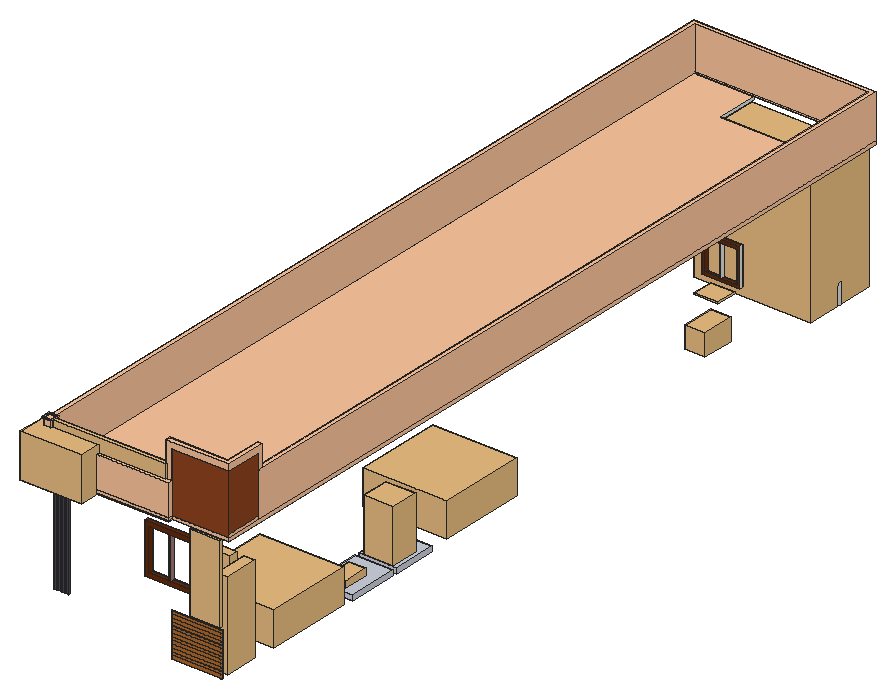
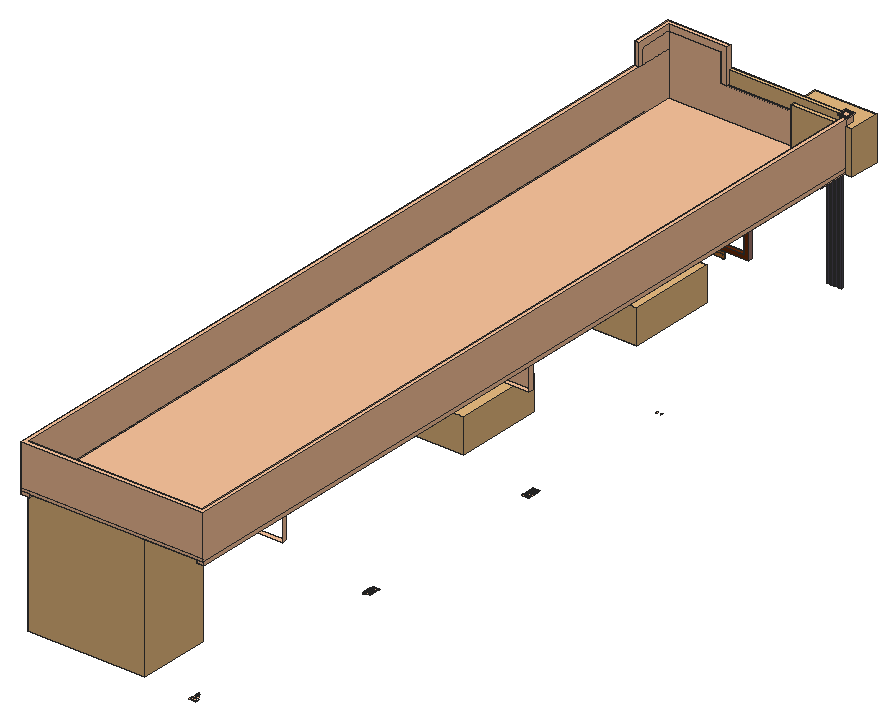
# SketchUp Ruby script. Lengths in inches.
U = 1.inch
M = Sketchup.active_model
def pt(a) = Geom::Point3d.new(a.map { |v| v * U })
def face(e, loops, mat)
  f = e.add_face(loops[0].map { |a| pt(a) })
  loops[1..].each { |l| e.add_face(l.map { |a| pt(a) }).erase! }
  f.material = f.back_material = mat if mat
  f
end
# faces: each face lists its corners as indices into pts; further lists are holes
def faces(e, pts, list, mat = nil) = list.each { |f| face(e, (f[0].is_a?(Array) ? f : [f]).map { |l| l.map { |i| pts[i] } }, mat) }
# xy, xz, yz: faces in a plane at the given z, y or x. An outline is a flat list of corners, or four numbers for a rectangle; further outlines are holes
def ring(l) = l.size == 4 ? [[l[0], l[1]], [l[2], l[1]], [l[2], l[3]], [l[0], l[3]]] : l.each_slice(2).to_a
def flat(e, list, mat, &to3) = list.each { |f| face(e, (f[0].is_a?(Array) ? f : [f]).map { |l| ring(l).map { |u, v| to3.(u, v) } }, mat) }
def xy(e, z, list, mat = nil) = flat(e, list, mat) { |x, y| [x, y, z] }
def xz(e, y, list, mat = nil) = flat(e, list, mat) { |x, z| [x, y, z] }
def yz(e, x, list, mat = nil) = flat(e, list, mat) { |y, z| [x, y, z] }
def lines(e, pts, list) = list.each { |a, b| e.add_line(pt(pts[a]), pt(pts[b])) }
# prism: a flat outline (further loops are holes) pulled along v
def prism(e, loops, v, mat = nil)
  f = face(e, loops, mat); d = Geom::Vector3d.new(v.map { |x| x * U })
  f.pushpull(f.normal.samedirection?(d) ? d.length : -d.length)
end
def box(e, o, s, mat = nil) = prism(e, [[o, [o[0] + s[0], o[1], o[2]], [o[0] + s[0], o[1] + s[1], o[2]], [o[0], o[1] + s[1], o[2]]]], [0, 0, s[2]], mat)
def at(x, y, z, deg = 0) = Geom::Transformation.translation(pt([x, y, z])) * Geom::Transformation.rotation(ORIGIN, Z_AXIS, deg.degrees)
def axes(o, x, y, z) = Geom::Transformation.new([*x, 0, *y, 0, *z, 0, *pt(o).to_a, 1])
def part(name) = M.definitions.add(name)
# library, detail: a bought-in or finely detailed component or shape, given as its bounding box
def library(name, o, s) = part(name).tap { |d| box(d.entities, o, s) }
def detail(e, o, s) = box(e.add_group.entities, o, s)
def put(e, d, t, mat = nil) = e.add_instance(d, t).tap { |i| i.material = mat if mat }
def group(e, t, mat = nil) = e.add_group.tap { |g| g.transformation = t; g.material = mat if mat }.entities
root = M.entities
M.materials.add("[0023_FireBrick]").color = [178, 34, 34]
M.materials.add("[Color A01]1").color = [163, 122, 112]
M.materials.add("[Color A02]1").color = [252, 197, 157]
M.materials.add("[Color M06]").color = [77, 72, 86]
M.materials.add("[Marble Carrara Floor Tile]").color = [204, 208, 219]
M.materials.add("[Wood Bamboo]").color = [177, 105, 43]
M.materials.add("[Wood Fence]1").color = [142, 67, 30]
M.materials.add("[Wood Veneer 02]").color = [107, 42, 7]
c1 = part("Group\#210")
box(c1.entities,[0,0,-0.3125],[36.0625,48,5.3125])
c2 = library("Group\#15",[-0.01,-1.53,0.79],[112.05,69.48,120])
c3 = library("Double bed",[0,0,0],[90.55,83.75,32.69])
c4 = part("Component\#5")
box(c4.entities,[0,-0.625,0],[48.6875,0.625,3.09])
c5 = library("P2 Single Open Right",[0,0,0],[8.91,82.42,82.52])
c6 = library("Group\#135",[0,0,0],[10.8125,33,84])
c7 = library("Squat+Toilet",[-7.87,-3.06,-5.41],[15.8,23.9,6.66])
c8 = library("My Toilet",[37.42,56.99,0],[19.17,25.6,30.6])
c9 = part("Frame upright")
box(c9.entities,[0,0,-39.22],[3.05,1.4,102],"[Color M06]")
c10 = library("Kitchen sink",[0,-0.57,-6.81],[19.24,30.87,20.8])
c11 = library("2-TABLE DE CUISSON CLC2",[-11.42,-10.04,0],[22.84,20.08,1.26])
c12 = part("Group87\#1")
xy(c12.entities,0,[[[-24,-24,24,24],[0.59,-20.0625,20.0625,20.0625],[-20.0625,-20.0625,-0.59,20.0625]]],"[Wood Veneer 02]")
xy(c12.entities,5.875,[[[-24,-24,24,24],[0.59,-20.0625,20.0625,20.0625],[-20.0625,-20.0625,-0.59,20.0625]]],"[Wood Veneer 02]")
xz(c12.entities,-24,[[-24,0,24,5.875]])
xz(c12.entities,-20.0625,[[-20.0625,0,-0.59,5.875],[0.59,0,20.0625,5.875]],"[Wood Veneer 02]")
xz(c12.entities,20.0625,[[-20.0625,0,-0.59,5.875],[0.59,0,20.0625,5.875]])
xz(c12.entities,24,[[-24,0,24,5.875]],"[Wood Veneer 02]")
yz(c12.entities,-24,[[-24,0,24,5.875]])
yz(c12.entities,-20.0625,[[-20.0625,0,20.0625,5.875]],"[Wood Veneer 02]")
yz(c12.entities,-0.59,[[-20.0625,0,20.0625,5.875]],"[Wood Veneer 02]")
yz(c12.entities,0.59,[[-20.0625,0,20.0625,5.875]])
yz(c12.entities,20.0625,[[-20.0625,0,20.0625,5.875]],"[Wood Veneer 02]")
yz(c12.entities,24,[[-24,0,24,5.875]])
c13 = library("jali",[235.9375,0,0],[159,318,2])
c14 = library("ARTIFICIAL VINES & FLOWERS",[-442.26,-138.3125,250.52],[58.45,28.9,41.46])
c15 = part("Square post")
box(c15.entities,[0,0,0],[7.1875,7.1875,27.41])
c16 = part("Component\#11")
xy(c16.entities,0,[[0,0,7.1875,7.1875]])
xy(c16.entities,12.79,[[[-0.9,-0.9,8.09,8.09],[0,0,7.1875,7.1875]],[0,0,7.1875,7.1875]])
xy(c16.entities,13.54,[[[-0.9,-0.9,8.09,8.09],[0,0,7.1875,7.1875]]])
xz(c16.entities,-0.9,[[-0.9,12.79,8.09,13.54]])
xz(c16.entities,0,[[0,0,7.1875,12.79],[0,12.79,7.1875,13.54]])
xz(c16.entities,7.1875,[[0,0,7.1875,12.79],[0,12.79,7.1875,13.54]])
xz(c16.entities,8.09,[[-0.9,12.79,8.09,13.54]])
yz(c16.entities,-0.9,[[-0.9,12.79,8.09,13.54]])
yz(c16.entities,0,[[0,0,7.1875,12.79],[0,12.79,7.1875,13.54]])
yz(c16.entities,7.1875,[[0,0,7.1875,12.79],[0,12.79,7.1875,13.54]])
yz(c16.entities,8.09,[[-0.9,12.79,8.09,13.54]])
c17 = library("Group\#181",[0,0,0],[107.67,3.9375,12.79])
box(root,[98.75,741.65,131.89],[75.61,3.31,19.68])
xy(root,131.89,[[11.25,222.37,12.14,223.25,11.26,224.13,10.36,223.26],[15.65,223.28,15.84,223.47,15.84,224.86,15.65,225.05,14.77,224.16],[15.84,224.86,15.84,225.24,15.65,225.05],[8.88,372.26,9.13,372.26,9.51,372.64,8.88,373.27],[9.13,372.26,9.89,372.26,9.51,372.64],
  [9.89,372.26,10.9,372.26,11.28,372.64,10.4,373.52,9.51,372.64],[10.9,372.26,11.66,372.26,11.28,372.64],[11.66,372.26,12.42,372.26,12.42,373.27,12.17,373.52,11.28,372.64],[12.42,372.26,12.68,372.26,13.06,372.64,12.42,373.27],[12.68,372.26,13.4375,372.26,13.06,372.64],
  [13.4375,372.26,14.45,372.26,14.83,372.64,13.94,373.52,13.06,372.64],[14.45,372.26,15.21,372.26,14.83,372.64],[15.21,372.26,15.84,372.26,15.84,373.27,15.65,373.46,14.83,372.64],[11.28,372.64,12.17,373.52,11.28,374.41,10.4,373.52],[13.06,372.64,13.94,373.52,13.06,374.41,12.42,373.78,12.42,373.27],
  [14.83,372.64,15.65,373.46,14.78,374.36,13.94,373.52],[12.42,373.27,12.42,373.78,12.17,373.52],[15.84,373.27,15.84,373.65,15.65,373.46],[15.65,373.46,15.84,373.65,15.84,375.04,15.65,375.23,14.78,374.36],[10.4,373.52,11.28,374.41,10.4,375.3,9.51,374.41],
  [12.17,373.52,12.42,373.78,12.42,375.04,12.17,375.3,11.28,374.41],[13.94,373.52,14.78,374.36,13.9,375.25,13.06,374.41],[8.88,373.78,9.51,374.41,8.88,375.04],[12.42,373.78,13.06,374.41,12.42,375.04],[14.78,374.36,15.65,375.23,14.78,376.13,13.9,375.25],
  [9.51,374.41,10.4,375.3,9.51,376.18,8.88,375.55,8.88,375.04],[11.28,374.41,12.17,375.3,11.28,376.18,10.4,375.3],[13.06,374.41,13.9,375.25,13.02,376.14,12.42,375.55,12.42,375.04],[12.42,375.04,12.42,375.55,12.17,375.3],[15.84,375.04,15.84,375.42,15.65,375.23],
  [15.65,375.23,15.84,375.42,15.84,376.82,15.65,377.01,14.78,376.13],[13.9,375.25,14.78,376.13,13.9,377.02,13.02,376.14],[10.4,375.3,11.28,376.18,10.4,377.07,9.51,376.18],[12.17,375.3,12.42,375.55,12.42,376.75,12.14,377.04,11.28,376.18],[8.88,375.55,9.51,376.18,8.88,376.82],
  [12.42,375.55,13.02,376.14,12.42,376.75],[14.78,376.13,15.65,377.01,14.78,377.9,13.9,377.02],[9.51,376.18,10.4,377.07,9.51,377.95,8.88,377.32,8.88,376.82],[11.28,376.18,12.14,377.04,11.26,377.93,10.4,377.07],[15.65,377.01,15.84,377.19,15.84,378.59,15.65,378.78,14.78,377.9],
  [13.9,377.02,14.78,377.9,13.9,378.8,13.02,377.92],[12.14,377.04,12.42,377.32,12.42,378.52,12.14,378.8125,11.26,377.93],[10.4,377.07,11.26,377.93,10.38,378.83,9.51,377.95],[8.88,377.32,9.51,377.95,8.88,378.59],[12.42,377.32,13.02,377.92,12.42,378.52],
  [14.78,377.9,15.65,378.78,14.78,379.67,13.9,378.8],[13.02,377.92,13.9,378.8,13.02,379.69,12.42,379.09,12.42,378.52],[11.26,377.93,12.14,378.8125,11.26,379.71,10.38,378.83],[9.51,377.95,10.38,378.83,9.51,379.72,8.88,379.09,8.88,378.59],[15.65,378.78,15.84,378.97,15.84,380.36,15.66,380.55,14.78,379.67],
  [13.9,378.8,14.78,379.67,13.9,380.57,13.02,379.69],[12.14,378.8125,12.42,379.09,12.42,380.3,12.14,380.58,11.26,379.71],[10.38,378.83,11.26,379.71,10.38,380.6,9.51,379.72],[8.88,379.09,9.51,379.72,8.88,380.36],[12.42,379.09,13.02,379.69,12.42,380.3],
  [14.78,379.67,15.66,380.55,14.78,381.45,13.9,380.57],[9.51,379.72,10.38,380.6,9.51,381.49,8.88,380.87,8.88,380.36],[13.9,380.57,14.78,381.45,13.91,382.35,13.02,381.46],[12.14,380.58,12.42,380.87,12.42,382.07,12.14,382.36,11.26,381.48],[14.78,381.45,15.66,382.33,14.79,383.23,13.91,382.35],
  [13.02,381.46,13.91,382.35,13.03,383.25,12.42,382.64,12.42,382.07],[12.42,382.07,12.42,382.64,12.14,382.36],[15.66,382.33,15.84,382.51,15.84,383.91,15.66,384.11,14.79,383.23],[13.91,382.35,14.79,383.23,13.92,384.14,13.03,383.25],[12.14,382.36,12.42,382.64,12.42,383.87,12.16,384.14,11.27,383.25],
  [10.38,382.37,11.27,383.25,10.39,384.15,9.51,383.27],[12.42,382.64,13.03,383.25,12.42,383.87],[14.79,383.23,15.66,384.11,14.82,385.03,13.92,384.14],[11.27,383.25,12.16,384.14,11.28,385.04,10.39,384.15],[13.03,383.25,13.92,384.14,13.05,385.04,12.42,384.41,12.42,383.87],
  [9.51,383.27,10.39,384.15,9.51,385.04,8.88,384.41,8.88,383.91],[12.42,383.87,12.42,384.41,12.16,384.14],[15.66,384.11,15.84,384.29,15.84,385.3,15.08,385.3,14.82,385.03],[12.16,384.14,12.42,384.41,12.42,385.3,11.54,385.3,11.28,385.04],[13.92,384.14,14.82,385.03,14.58,385.3,13.31,385.3,13.05,385.04],
  [10.39,384.15,11.28,385.04,11.03,385.3,9.76,385.3,9.51,385.04],[8.88,384.41,9.51,385.04,9.26,385.3,8.88,385.3],[12.42,384.41,13.05,385.04,12.8,385.3,12.42,385.3],[8.88,564.35,9.13,564.35,9.51,564.73,8.88,565.36],[9.13,564.35,9.89,564.35,9.51,564.73],
  [9.89,564.35,10.9,564.35,11.28,564.73,10.4,565.62,9.51,564.73],[10.9,564.35,11.66,564.35,11.28,564.73],[11.66,564.35,12.42,564.35,12.42,565.36,12.17,565.62,11.28,564.73],[12.42,564.35,12.68,564.35,13.06,564.73,12.42,565.36],[12.68,564.35,13.4375,564.35,13.06,564.73],
  [13.4375,564.35,14.45,564.35,14.83,564.73,13.94,565.62,13.06,564.73],[14.45,564.35,15.21,564.35,14.83,564.73],[9.51,564.73,10.4,565.62,9.51,566.5,8.88,565.87,8.88,565.36],[11.28,564.73,12.17,565.62,11.28,566.5,10.4,565.62],[13.06,564.73,13.94,565.62,13.06,566.5,12.42,565.87,12.42,565.36],
  [13.94,565.62,14.78,566.45,13.9,567.34,13.06,566.5],[8.88,565.87,9.51,566.5,8.88,567.14],[12.42,565.87,13.06,566.5,12.42,567.14],[14.78,566.45,15.65,567.33,14.77,568.21,13.9,567.34],[9.51,566.5,10.4,567.39,9.51,568.28,8.88,567.64,8.88,567.14],
  [13.06,566.5,13.9,567.34,13.02,568.24,12.42,567.64,12.42,567.14],[15.65,567.33,15.84,567.52,15.84,568.91,15.65,569.1,14.77,568.21],[13.9,567.34,14.77,568.21,13.88,569.1,13.02,568.24],[10.4,567.39,11.28,568.28,10.4,569.16,9.51,568.28],[12.17,567.39,12.42,567.64,12.42,568.85,12.14,569.13,11.28,568.28],
  [8.88,567.64,9.51,568.28,8.88,568.91],[12.42,567.64,13.02,568.24,12.42,568.85],[14.77,568.21,15.65,569.1,14.77,569.99,13.88,569.1],[13.02,568.24,13.88,569.1,12.99,569.99,12.42,569.42,12.42,568.85],[9.51,568.28,10.4,569.16,9.51,570.05,8.88,569.42,8.88,568.91],
  [11.28,568.28,12.14,569.13,11.26,570.03,10.4,569.16],[12.42,568.85,12.42,569.42,12.14,569.13],[13.88,569.1,14.77,569.99,13.88,570.87,12.99,569.99],[15.65,569.1,15.84,569.29,15.84,570.68,15.65,570.87,14.77,569.99],[12.14,569.13,12.42,569.42,12.42,570.56,12.11,570.87,11.26,570.03],
  [10.4,569.16,11.26,570.03,10.38,570.92,9.51,570.05],[8.88,569.42,9.51,570.05,8.88,570.68],[12.42,569.42,12.99,569.99,12.42,570.56],[12.99,569.99,13.88,570.87,12.99,571.76,12.42,571.1875,12.42,570.56],[14.77,569.99,15.65,570.87,14.77,571.76,13.88,570.87],
  [11.26,570.03,12.11,570.87,11.22,571.76,10.38,570.92],[9.51,570.05,10.38,570.92,9.51,571.81,8.88,571.1875,8.88,570.68],[12.11,570.87,12.42,571.1875,12.42,572.33,12.11,572.65,11.22,571.76],[13.88,570.87,14.77,571.76,13.88,572.65,12.99,571.76],[10.38,570.92,11.22,571.76,10.35,572.63,9.51,571.81],
  [8.88,571.1875,9.51,571.81,8.88,572.46],[12.42,571.1875,12.99,571.76,12.42,572.33],[11.22,571.76,12.11,572.65,11.25,573.51,10.35,572.63],[12.99,571.76,13.88,572.65,12.99,573.53,12.42,572.96,12.42,572.33],[14.77,571.76,15.65,572.65,14.77,573.53,13.88,572.65],
  [9.51,571.81,10.35,572.63,9.46,573.52,8.88,572.96,8.88,572.46],[12.42,572.33,12.42,572.96,12.11,572.65],[10.35,572.63,11.25,573.51,10.36,574.4,9.46,573.52],[12.11,572.65,12.42,572.96,12.42,574.1,12.14,574.38,11.25,573.51],[13.88,572.65,14.77,573.53,13.88,574.42,12.99,573.53],
  [15.65,572.65,15.84,572.84,15.84,574.23,15.65,574.42,14.77,573.53],[8.88,572.96,9.46,573.52,8.88,574.1],[12.42,572.96,12.99,573.53,12.42,574.1],[11.25,573.51,12.14,574.38,11.26,575.27,10.36,574.4],[9.46,573.52,10.36,574.4,9.46,575.29,8.88,574.73,8.88,574.1],
  [12.99,573.53,13.88,574.42,13.04,575.26,12.42,574.66,12.42,574.1],[14.77,573.53,15.65,574.42,14.77,575.3,13.88,574.42],[12.42,574.1,12.42,574.66,12.14,574.38],[12.14,574.38,12.42,574.66,12.42,575.875,12.15,576.14,11.26,575.27],[13.88,574.42,14.77,575.3,13.93,576.14,13.04,575.26],
  [15.65,574.42,15.84,574.61,15.84,576,15.65,576.19,14.77,575.3],[12.42,574.66,13.04,575.26,12.42,575.875],[13.04,575.26,13.93,576.14,13.05,577.02,12.42,576.41,12.42,575.875],[14.77,575.3,15.65,576.19,14.83,577.02,13.93,576.14],[13.93,576.14,14.83,577.02,14.58,577.27,13.31,577.27,13.05,577.02],
  [15.84,771.51,15.84,771.89,15.66,771.7],[15.66,771.7,15.84,771.89,15.84,773.29,15.66,773.47,14.79,772.57],[15.84,773.29,15.84,773.67,15.66,773.47],[13.91,773.45,14.78,774.35,13.94,775.1875,13.06,774.3],[15.66,773.47,15.84,773.67,15.84,775.06,15.66,775.25,15.84,775.44,15.84,776.83,15.72,776.96,14.83,776.07,15.66,775.25,14.78,774.35],
  [15.84,775.06,15.84,775.44,15.66,775.25],[15.84,776.83,15.84,777.09,15.72,776.96],[12.17,776.96,13.06,777.85,12.17,778.73,11.28,777.85],[13.94,776.96,14.83,777.85,15.72,778.73,14.83,779.62,15.66,780.45,14.79,781.35,13.94,780.51,13.06,781.39,13.92,782.25,13.05,783.16,13.92,782.25,14.79,781.35,13.94,780.51,15.84,778.61,15.84,777.09,15.72,776.96,14.83,777.85,13.94,778.73,13.06,777.85],[15.72,776.96,15.84,777.09,15.84,778.61,15.72,778.73,14.83,777.85],
  [15.84,778.61,15.84,778.86,15.72,778.73],[13.06,779.62,13.94,780.51,12.17,782.28,11.28,783.16,9.51,781.39,8.88,782.02,8.88,780.76,10.4,782.28,11.28,781.39,13.05,783.16,13.92,782.25,14.82,783.15,14.58,783.42,13.31,783.42,12.17,782.28,13.06,781.39,12.17,780.51],[15.84,780.25,15.84,780.63,15.66,780.45],[15.66,782.22,15.84,782.4,15.84,783.42,15.08,783.42,14.82,783.15],[9.51,783.16,9.76,783.42,9.26,783.42],
  [11.28,783.16,11.54,783.42,11.03,783.42],[13.05,783.16,13.31,783.42,12.8,783.42]],"[Color A02]1")
xy(root,167.89,[[104.48,665.91,140.48,670.34]],"[Color A02]1")
xy(root,203.89,[[104.48,665.91,140.48,670.34]],"[Color A02]1")
xy(root,215.89,[[126.53,46.0625,150.53,50.62],[52.9375,119.63,57.37,155.6],[82.95,164.21,87.38,194.22],[57.37,258.67,77.375,263.23],[16.86,371.24,52.9375,375.68],
  [57.37,371.24,83.33,375.68],[96.37,573.85,126.38,578.28],[16.86,665.91,64.84,670.34]],"[Color A02]1")
xy(root,251.89,[[0.9,46.0625,7.87,784.43],[52.9375,46.0625,156.53,46.0625,156.53,50.62,57.37,50.62,57.37,119.63,52.9375,119.63],[156.53,46.0625,166.9,50.62],[171.33,61,175.89,61,175.89,212.21,171.33,212.21,171.33,164.21,52.9375,164.21,52.9375,119.63,57.37,119.63,57.37,160.15,171.33,160.15],[82.95,164.21,87.38,164.21,87.38,212.2,166.89,212.2,166.89,216.63,57.37,216.63,57.37,375.68,16.86,375.68,16.86,371.24,52.9375,371.24,52.9375,212.2,82.95,212.2],
  [171.33,227.14,175.89,227.14,175.89,371.25,171.33,371.25,171.33,263.23,57.37,263.23,57.37,258.67,171.33,258.67],[57.37,371.24,166.9,375.68],[7.87,386.1875,12.42,563.34],[171.33,386.1875,175.89,563.34],[87.89,573.85,166.9,573.85,166.9,578.28,92.44,578.28,92.44,665.91,171.33,665.91,171.33,578.28,175.89,578.28,175.89,670.34,16.86,670.34,16.86,665.91,87.89,665.91],
  [7.87,578.28,12.42,578.28,12.42,665.91,16.86,665.91,16.86,670.34,7.87,670.34]],"[Color A02]1")
xz(root,371.24,[[16.86,215.89,52.9375,251.89]],"[Color A02]1")
yz(root,16.86,[[371.24,215.89,375.68,251.89],[665.91,215.89,670.34,251.89]],"[Color A02]1")
yz(root,104.48,[[665.91,167.89,670.34,203.89]],"[Color A02]1")
yz(root,140.48,[[665.91,167.89,670.34,203.89]],"[Color A02]1")
p = [[169.9,779.32,257.89],[6.9,779.32,257.89],[169.9,46.0625,257.89],[175.89,785.32,257.89],[0.9,785.32,257.89],[107.4375,669.12,170.88],
  [122.04,669.12,170.88],[110.75,50.62,171.82],[110.75,50.62,211.95],[91.28,50.62,171.82],[91.28,50.62,211.95],[70.625,50.62,211.95],
  [70.625,50.62,171.82],[90.09,50.62,211.95],[90.09,50.62,171.82]]
lines(root,p,[[0,1],[2,0],[3,4],[5,6],[7,8],[9,7],[10,9],[8,10],[11,12],[13,11],[14,13],[12,14]])
put(root,c1,at(135.46,164.2,132.2),"[Marble Carrara Floor Tile]")
put(root,c1,axes([135.46,216.63,132.2],[1,0,0],[0,0.87583,0],[0,0,1]),"[Marble Carrara Floor Tile]")
put(root,c2,at(62.29,710.41,131.1))
put(root,c3,axes([167.8125,281.22,132.26],[-0.89,0,0],[0,1,0],[0,0,1]))
put(root,c3,axes([171.125,70.44,132.26],[-0.89,0,0],[0,1,0],[0,0,1]))
put(root,c4,at(121.89,10.0625,132.5),"[Wood Bamboo]")
put(root,c5,axes([150.59,43.27,133.39],[0,1,0],[-0.3,0,0],[0,0,1]))
put(root,c6,at(161.9,13.0625,135.04))
put(root,c4,at(121.89,10.0625,135.68),"[Wood Bamboo]")
put(root,c7,at(153.05,171.69,142.3))
put(root,c8,axes([223.82,302.41,137.85],[-1.48104,0,0],[0,-1.04,0],[0,0,1.65]))
put(root,c4,at(121.89,10.0625,138.87),"[Wood Bamboo]")
put(root,c4,at(121.89,10.0625,142.06),"[Wood Bamboo]")
put(root,c4,at(121.89,10.0625,145.25),"[Wood Bamboo]")
put(root,c4,at(121.89,10.0625,148.43),"[Wood Bamboo]")
g1 = group(root,at(5.65,14.01,149.89))
put(g1,c9,at(0,0,39.22))
put(g1,c9,at(3.75,0,39.22))
put(g1,c9,at(11.4375,0,39.22))
put(g1,c9,at(7.5,0,39.22))
put(root,c4,at(121.89,10.0625,151.62),"[Wood Bamboo]")
put(root,c4,at(121.89,10.0625,154.81),"[Wood Bamboo]")
put(root,c10,at(152.21,586.64,162.18))
put(root,c4,at(121.89,10.0625,158),"[Wood Bamboo]")
put(root,c4,at(121.89,10.0625,161.18),"[Wood Bamboo]")
put(root,c11,at(123.65,656.6875,161.89))
put(root,c4,at(121.89,10.0625,164.37),"[Wood Bamboo]")
put(root,c4,at(121.89,10.0625,167.56),"[Wood Bamboo]")
put(root,c12,axes([90.6875,50.62,191.89],[1,0,0],[0,0,1],[0,-0.72,0]),"[Color A01]1")
put(root,c12,axes([122.48,669.12,186.125],[0.75,0,0],[0,0,0.76],[0,-0.5472,0]))
put(root,c4,at(121.89,10.0625,170.73),"[Wood Bamboo]")
put(root,c13,axes([98.13,9.125,176.82],[0.18169,0,0],[0,0,0.23605],[0,-1.01,0]))
put(root,c14,at(436.24,126.71,0))
g2 = group(root,at(0.88,6.0625,0))
g3 = group(g2,at(0,0,0))
xy(g3,251.07,[[0.01,0,0.01,40,15.96,40,15.96,728.43,26.63,728.43,26.63,10.67,110.33,10.67,110.33,29.33,41.375,29.33,41.375,728.43,52.04,728.43,52.04,40,121,40,121,0]],"[Color A02]1")
xy(g3,251.89,[[0.01,0,121,0,121,40,52.04,40,52.04,728.43,41.375,728.43,41.375,29.33,110.33,29.33,110.33,10.67,26.63,10.67,26.63,728.43,15.96,728.43,15.96,40,0.01,40],[121,4,121,40,52.04,40,52.04,728.43,61.39,728.43,61.39,734.68,131.41,734.68,131.41,774.75,166.24,774.75,166.24,779.25,175.01,779.25,175.01,4],[0,24.89,0.01,40],[0.01,40,0.01,778.37,6.96,778.37,6.96,774.75,61.39,774.75,61.39,728.43,15.96,728.43,15.96,40]],"[Color A02]1")
xy(g3,253.01,[[26.63,10.67,26.63,728.43,41.375,728.43,41.375,29.33,110.33,29.33,110.33,10.67]],"[0023_FireBrick]")
xy(g3,255.07,[[0.01,0,121,0,121,4,175.01,4,175.01,779.25,166.24,779.25,166.24,774.75,131.41,774.75,131.41,734.68,61.39,734.68,61.39,774.75,6.96,774.75,6.96,778.37,0.01,778.37]],"[Color A02]1")
xz(g3,0,[[0.01,251.07,121,251.89],[0.01,251.89,121,255.07]],"[Color A02]1")
xz(g3,4,[[121,251.89,175.01,255.07]],"[Color A02]1")
xz(g3,10.67,[[26.63,251.07,110.33,251.89],[26.63,251.89,110.33,253.01]],"[Color A02]1")
xz(g3,29.33,[[41.375,251.07,110.33,251.89],[41.375,251.89,110.33,253.01]],"[Color A02]1")
xz(g3,40,[[0.01,251.07,15.96,251.89],[52.04,251.07,121,251.89]],"[Color A02]1")
xz(g3,728.43,[[26.63,251.89,41.375,253.01],[41.375,251.89,61.39,253.01]])
xz(g3,728.43,[[15.96,251.07,26.63,251.89],[26.63,251.07,41.375,251.89],[41.375,251.07,52.04,251.89]],"[Color A02]1")
xz(g3,734.68,[[61.39,251.89,131.41,255.07]])
xz(g3,774.75,[[131.41,251.89,166.24,255.07]])
xz(g3,774.75,[[6.96,251.89,61.39,255.07]],"[Color A02]1")
xz(g3,778.37,[[0.01,251.89,6.96,255.07]],"[Color A02]1")
xz(g3,779.25,[[166.24,251.89,175.01,255.07]],"[Color A02]1")
yz(g3,0.01,[[0,251.07,24.89,251.89],[24.89,251.07,40,251.89],[0,251.89,778.37,255.07]],"[Color A02]1")
yz(g3,6.96,[[774.75,251.89,778.37,255.07]],"[Color A02]1")
yz(g3,15.96,[[40,251.07,728.43,251.89]],"[Color A02]1")
yz(g3,26.63,[[10.67,251.07,728.43,251.89],[10.67,251.89,728.43,253.01]],"[Color A02]1")
yz(g3,41.375,[[29.33,251.07,728.43,251.89],[29.33,251.89,728.43,253.01]],"[Color A02]1")
yz(g3,52.04,[[40,251.07,728.43,251.89]],"[Color A02]1")
yz(g3,61.39,[[728.43,251.89,734.68,253.01],[734.68,251.89,774.75,255.07]])
yz(g3,110.33,[[10.67,251.07,29.33,251.89],[10.67,251.89,29.33,253.01]],"[Color A02]1")
yz(g3,121,[[0,251.07,4,251.89],[4,251.07,40,251.89],[0,251.89,4,255.07]],"[Color A02]1")
yz(g3,131.41,[[734.68,251.89,774.75,255.07]])
yz(g3,166.24,[[774.75,251.89,779.25,255.07]],"[Color A02]1")
yz(g3,175.01,[[4,251.89,779.25,255.07]],"[Color A02]1")
put(root,c15,at(0.9,6.0625,255.07),"[Color A02]1")
g4 = group(root,at(0.9,6.0625,255.07))
xy(g4,0,[[[39.17,0,39.17,4,0,4,0,779.25,174.99,779.25,174.99,4,120.99,4,120.99,0],[4.5,8.5,170.5,774.75]]],"[Color A02]1")
xy(g4,27.41,[[0,0,39.17,4]],"[Color A02]1")
xy(g4,30.125,[[0,0,120.99,0,120.99,4,114.99,4,114.99,8.5,0,8.5],[114.99,4,120.99,8.5]],"[Color A02]1")
xy(g4,42.125,[[0,8.5,4.5,8.5,4.5,774.75,170.5,774.75,170.5,44.375,174.99,44.375,174.99,779.25,0,779.25]],"[Color A02]1")
xy(g4,57.05,[[120.99,4,174.99,4,174.99,40,170.5,40,170.5,8.5,120.99,8.5]],"[Color A02]1")
xy(g4,63.05,[[114.99,4,174.99,4,174.99,44.375,170.5,44.375,170.5,8.5,114.99,8.5]],"[Color A02]1")
xz(g4,0,[[39.17,0,120.99,30.125],[0,27.41,39.17,30.125]],"[Color A02]1")
xz(g4,4,[[0,0,39.17,27.41],[114.99,30.125,120.99,30.125,120.99,57.05,174.99,57.05,174.99,63.05,114.99,63.05]],"[Color A02]1")
xz(g4,4,[[120.99,0,174.99,57.05]],"[Wood Fence]1")
xz(g4,8.5,[[4.5,0,4.5,30.125,120.99,30.125,120.99,57.05,170.5,57.05,170.5,0],[0,30.125,4.5,42.125],[114.99,30.125,114.99,63.05,170.5,63.05,170.5,57.05,120.99,57.05,120.99,30.125]],"[Color A02]1")
xz(g4,40,[[170.5,42.125,174.99,57.05]],"[Color A02]1")
xz(g4,44.375,[[170.5,42.125,174.99,63.05]],"[Color A02]1")
xz(g4,774.75,[[4.5,0,170.5,42.125]],"[Color A02]1")
xz(g4,779.25,[[0,0,174.99,42.125]],"[Color A02]1")
yz(g4,0,[[4,0,4,27.41,0,27.41,0,30.125,8.5,30.125,8.5,42.125,779.25,42.125,779.25,0]],"[Color A02]1")
yz(g4,4.5,[[8.5,0,774.75,42.125]],"[Color A02]1")
yz(g4,39.17,[[0,0,4,27.41]],"[Color A02]1")
yz(g4,114.99,[[4,30.125,8.5,63.05]],"[Color A02]1")
yz(g4,120.99,[[0,0,4,30.125],[4,30.125,8.5,57.05]],"[Color A02]1")
yz(g4,170.5,[[8.5,0,774.75,42.125],[40,42.125,40,57.05,8.5,57.05,8.5,63.05,44.375,63.05,44.375,42.125],[8.5,42.125,40,57.05]],"[Color A02]1")
yz(g4,174.99,[[4,0,40,2.8125],[40,0,779.25,42.125],[40,42.125,44.375,42.125,44.375,63.05,4,63.05,4,57.05,40,57.05]],"[Color A02]1")
yz(g4,174.99,[[4,2.8125,40,57.05]],"[Wood Fence]1")
put(root,c16,at(0.9,7.375,285.2),"[Color A02]1")
put(root,c17,axes([8.3,9,285.2],[1.01,0,0],[0,1,0],[0,0,1]))
